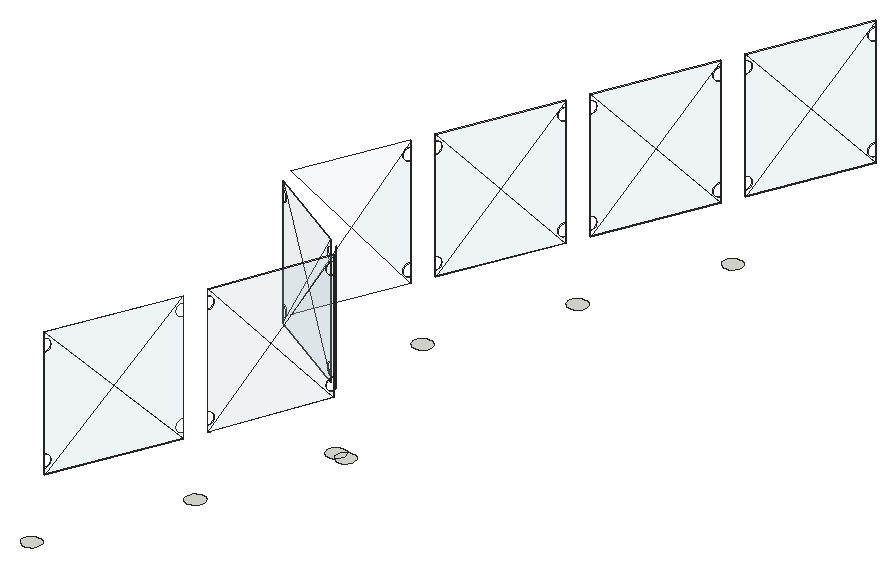
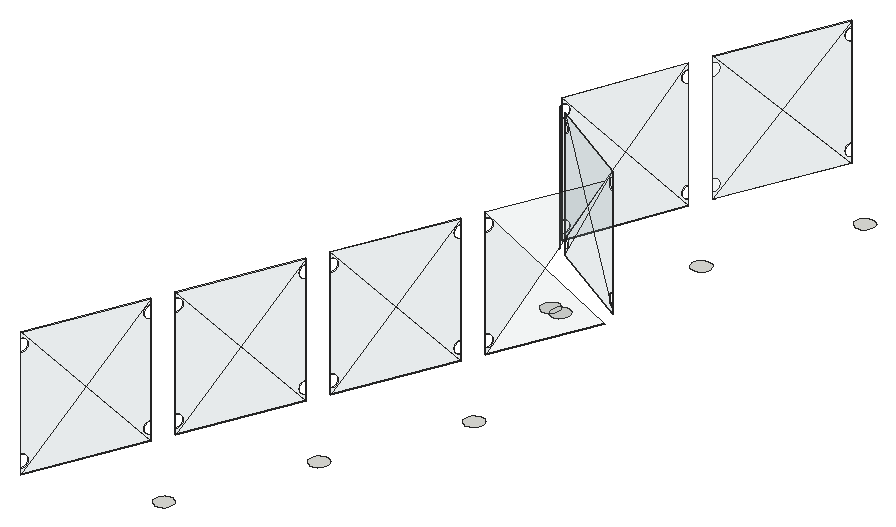
# SketchUp Ruby script. Lengths in inches.
U = 1.inch
M = Sketchup.active_model
def pt(a) = Geom::Point3d.new(a.map { |v| v * U })
def face(e, loops, mat)
  f = e.add_face(loops[0].map { |a| pt(a) })
  loops[1..].each { |l| e.add_face(l.map { |a| pt(a) }).erase! }
  f.material = f.back_material = mat if mat
  f
end
# faces: each face lists its corners as indices into pts; further lists are holes
def faces(e, pts, list, mat = nil) = list.each { |f| face(e, (f[0].is_a?(Array) ? f : [f]).map { |l| l.map { |i| pts[i] } }, mat) }
# xy, xz, yz: faces in a plane at the given z, y or x. An outline is a flat list of corners, or four numbers for a rectangle; further outlines are holes
def ring(l) = l.size == 4 ? [[l[0], l[1]], [l[2], l[1]], [l[2], l[3]], [l[0], l[3]]] : l.each_slice(2).to_a
def flat(e, list, mat, &to3) = list.each { |f| face(e, (f[0].is_a?(Array) ? f : [f]).map { |l| ring(l).map { |u, v| to3.(u, v) } }, mat) }
def xy(e, z, list, mat = nil) = flat(e, list, mat) { |x, y| [x, y, z] }
def xz(e, y, list, mat = nil) = flat(e, list, mat) { |x, z| [x, y, z] }
def yz(e, x, list, mat = nil) = flat(e, list, mat) { |y, z| [x, y, z] }
def lines(e, pts, list) = list.each { |a, b| e.add_line(pt(pts[a]), pt(pts[b])) }
# prism: a flat outline (further loops are holes) pulled along v
def prism(e, loops, v, mat = nil)
  f = face(e, loops, mat); d = Geom::Vector3d.new(v.map { |x| x * U })
  f.pushpull(f.normal.samedirection?(d) ? d.length : -d.length)
end
def box(e, o, s, mat = nil) = prism(e, [[o, [o[0] + s[0], o[1], o[2]], [o[0] + s[0], o[1] + s[1], o[2]], [o[0], o[1] + s[1], o[2]]]], [0, 0, s[2]], mat)
def at(x, y, z, deg = 0) = Geom::Transformation.translation(pt([x, y, z])) * Geom::Transformation.rotation(ORIGIN, Z_AXIS, deg.degrees)
def axes(o, x, y, z) = Geom::Transformation.new([*x, 0, *y, 0, *z, 0, *pt(o).to_a, 1])
def part(name) = M.definitions.add(name)
# library, detail: a bought-in or finely detailed component or shape, given as its bounding box
def library(name, o, s) = part(name).tap { |d| box(d.entities, o, s) }
def detail(e, o, s) = box(e.add_group.entities, o, s)
def put(e, d, t, mat = nil) = e.add_instance(d, t).tap { |i| i.material = mat if mat }
def group(e, t, mat = nil) = e.add_group.tap { |g| g.transformation = t; g.material = mat if mat }.entities
root = M.entities
M.materials.add("Glass_Safety_01").color = [204, 235, 244]
M.materials["Glass_Safety_01"].alpha = 0.1
xy(root,321.858,[[963.534,810.319,963.937,810.401,964.305,810.585,964.612,810.858,964.838,811.202,964.968,811.592,964.993,812.002,964.91,812.405,964.726,812.772,964.453,813.08,964.11,813.306,963.72,813.436,963.309,813.46,962.906,813.377,962.539,813.193,962.231,812.92,962.005,812.577,961.875,812.187,961.851,811.777,961.934,811.374,962.118,811.006,962.391,810.699,962.734,810.473,963.124,810.343],[973.7,833.66,974.103,833.743,974.471,833.927,974.778,834.2,975.004,834.543,975.134,834.933,975.159,835.344,975.076,835.746,974.892,836.114,974.619,836.421,974.276,836.648,973.886,836.777,973.475,836.802,973.072,836.719,972.705,836.535,972.397,836.262,972.171,835.919,972.041,835.529,972.017,835.118,972.1,834.716,972.284,834.348,972.557,834.041,972.9,833.814,973.29,833.685],[982.568,855.712,982.97,855.795,983.338,855.979,983.645,856.252,983.872,856.595,984.002,856.985,984.026,857.396,983.943,857.799,983.759,858.166,983.486,858.474,983.143,858.7,982.753,858.83,982.343,858.854,981.94,858.771,981.708,858.655,981.901,858.437,982.085,858.07,982.168,857.667,982.143,857.256,982.014,856.866,981.787,856.523,981.48,856.25,981.345,856.182,981.424,856.093,981.767,855.867,982.157,855.737],[980.71,855.983,981.112,856.066,981.345,856.182,981.151,856.4,980.967,856.768,980.884,857.171,980.909,857.581,981.039,857.971,981.265,858.314,981.572,858.587,981.708,858.655,981.628,858.745,981.285,858.971,980.895,859.101,980.485,859.125,980.082,859.042,979.714,858.858,979.407,858.585,979.18,858.242,979.051,857.852,979.026,857.442,979.109,857.039,979.293,856.671,979.566,856.364,979.909,856.138,980.299,856.008],[981.345,856.182,981.48,856.25,981.787,856.523,982.014,856.866,982.143,857.256,982.168,857.667,982.085,858.07,981.901,858.437,981.708,858.655,981.572,858.587,981.265,858.314,981.039,857.971,980.909,857.581,980.884,857.171,980.967,856.768,981.151,856.4],
  [970.873,887.274,971.276,887.357,971.644,887.541,971.951,887.814,972.177,888.157,972.307,888.547,972.332,888.957,972.249,889.36,972.065,889.728,971.792,890.035,971.449,890.261,971.059,890.391,970.648,890.416,970.245,890.333,969.878,890.149,969.57,889.876,969.344,889.533,969.214,889.143,969.19,888.732,969.273,888.33,969.457,887.962,969.73,887.655,970.073,887.428,970.463,887.298],[980.502,909.381,980.904,909.464,981.272,909.648,981.579,909.921,981.806,910.264,981.935,910.654,981.96,911.064,981.877,911.467,981.693,911.835,981.42,912.142,981.077,912.368,980.687,912.498,980.276,912.522,979.874,912.44,979.506,912.256,979.199,911.983,978.972,911.64,978.843,911.249,978.818,910.839,978.901,910.436,979.085,910.069,979.358,909.761,979.701,909.535,980.091,909.405],[990.144,931.521,990.547,931.604,990.915,931.788,991.222,932.061,991.448,932.404,991.578,932.794,991.602,933.204,991.52,933.607,991.336,933.975,991.063,934.282,990.72,934.508,990.329,934.638,989.919,934.663,989.516,934.58,989.149,934.396,988.841,934.123,988.615,933.78,988.485,933.39,988.461,932.979,988.544,932.577,988.728,932.209,989.001,931.901,989.344,931.675,989.734,931.545]])
xy(root,331.897,[[964.298,813.655,964.118,813.733,972.953,833.526],[964.118,813.733,972.772,833.605,972.953,833.526],[974.413,837.021,974.231,837.094,981.873,855.571],[974.231,837.094,981.69,855.645,981.873,855.571],[980.493,857.47,980.489,857.471,980.517,857.665],
  [980.493,857.47,980.517,857.665,980.521,857.665],[978.839,858.444,963.309,867.306,963.406,867.477],[978.839,858.444,963.406,867.477,978.936,858.615],[962.68,870.044,962.499,870.122,970.134,887.159],[962.499,870.122,969.953,887.238,970.134,887.159],
  [971.637,890.61,971.457,890.689,979.757,909.255],[971.457,890.689,979.577,909.334,979.757,909.255],[981.265,912.717,981.085,912.796,989.4,931.395],[981.085,912.796,989.219,931.473,989.4,931.395],[990.908,934.857,990.727,934.936,999.017,953.477],
  [990.727,934.936,998.837,953.555,999.017,953.477]],"Glass_Safety_01")
xz(root,857.665,[[980.517,331.897,980.521,333]],"Glass_Safety_01")
p = [[964.118,813.733,331.897],[964.298,813.655,331.897],[964.298,813.655,333],[964.298,813.655,335.126],[964.298,813.655,351.283],[964.298,813.655,353.409],
  [964.298,813.655,354.511],[964.118,813.733,354.511],[964.118,813.733,353.409],[964.118,813.733,351.283],[964.118,813.733,335.126],[964.118,813.733,333],
  [964.227,813.986,333.036],[964.33,814.221,333.142],[964.418,814.423,333.311],[964.485,814.577,333.531],[964.528,814.675,333.787],[964.542,814.708,334.0625],
  [964.528,814.675,334.338],[964.485,814.577,334.594],[964.418,814.423,334.814],[964.33,814.221,334.983],[964.227,813.986,335.089],[964.227,813.986,351.319],
  [964.33,814.221,351.425],[964.418,814.423,351.594],[964.485,814.577,351.814],[964.528,814.675,352.071],[964.542,814.708,352.346],[964.528,814.675,352.621],
  [964.485,814.577,352.877],[964.418,814.423,353.098],[964.33,814.221,353.267],[964.227,813.986,353.373],[972.772,833.605,331.897],[972.772,833.605,354.511],
  [972.772,833.605,353.409],[972.772,833.605,351.283],[972.772,833.605,335.126],[972.772,833.605,333],[964.408,813.907,335.089],[964.51,814.142,334.983],
  [964.598,814.344,334.814],[964.666,814.499,334.594],[964.708,814.596,334.338],[964.723,814.629,334.0625],[964.708,814.596,333.787],[964.666,814.499,333.531],
  [964.598,814.344,333.311],[964.51,814.142,333.142],[964.408,813.907,333.036],[972.953,833.526,354.511],[964.408,813.907,353.373],[964.51,814.142,353.267],
  [964.598,814.344,353.098],[964.666,814.499,352.877],[964.708,814.596,352.621],[964.723,814.629,352.346],[964.708,814.596,352.071],[964.666,814.499,351.814],
  [964.598,814.344,351.594],[964.51,814.142,351.425],[964.408,813.907,351.319],[972.953,833.526,331.897],[972.953,833.526,333],[972.892,833.387,333],
  [972.782,833.135,333.036],[972.68,832.9,333.142],[972.592,832.698,333.311],[972.524,832.543,333.531],[972.482,832.446,333.787],[972.467,832.412,334.0625],
  [972.482,832.446,334.338],[972.524,832.543,334.594],[972.592,832.698,334.814],[972.68,832.9,334.983],[972.782,833.135,335.089],[972.892,833.387,335.126],
  [972.953,833.526,335.126],[972.953,833.526,351.283],[972.892,833.387,351.283],[972.782,833.135,351.319],[972.68,832.9,351.425],[972.592,832.698,351.594],
  [972.524,832.543,351.814],[972.482,832.446,352.071],[972.467,832.412,352.346],[972.482,832.446,352.621],[972.524,832.543,352.877],[972.592,832.698,353.098],
  [972.68,832.9,353.267],[972.782,833.135,353.373],[972.892,833.387,353.409],[972.953,833.526,353.409],[974.231,837.094,331.897],[974.413,837.021,331.897],
  [974.413,837.021,333],[974.413,837.021,335.126],[974.413,837.021,351.283],[974.413,837.021,353.409],[974.413,837.021,354.511],[974.231,837.094,354.511],
  [974.231,837.094,353.409],[974.231,837.094,351.283],[974.231,837.094,335.126],[974.231,837.094,333],[974.516,837.276,335.089],[974.612,837.514,334.983],
  [974.694,837.718,334.814],[974.757,837.875,334.594],[974.797,837.973,334.338],[974.81,838.007,334.0625],[974.797,837.973,333.787],[974.757,837.875,333.531],
  [974.694,837.718,333.311],[974.612,837.514,333.142],[974.516,837.276,333.036],[981.873,855.571,354.511],[974.516,837.276,353.373],[974.612,837.514,353.267],
  [974.694,837.718,353.098],[974.757,837.875,352.877],[974.797,837.973,352.621],[974.81,838.007,352.346],[974.797,837.973,352.071],[974.757,837.875,351.814],
  [974.694,837.718,351.594],[974.612,837.514,351.425],[974.516,837.276,351.319],[981.873,855.571,331.897],[981.873,855.571,333],[981.812,855.42,333],
  [981.709,855.165,333.036],[981.614,854.927,333.142],[981.532,854.723,333.311],[981.469,854.566,333.531],[981.429,854.468,333.787],[981.415,854.434,334.0625],
  [981.429,854.468,334.338],[981.469,854.566,334.594],[981.532,854.723,334.814],[981.614,854.927,334.983],[981.709,855.165,335.089],[981.812,855.42,335.126],
  [981.873,855.571,335.126],[981.873,855.571,351.283],[981.812,855.42,351.283],[981.709,855.165,351.319],[981.614,854.927,351.425],[981.532,854.723,351.594],
  [981.469,854.566,351.814],[981.429,854.468,352.071],[981.415,854.434,352.346],[981.429,854.468,352.621],[981.469,854.566,352.877],[981.532,854.723,353.098],
  [981.614,854.927,353.267],[981.709,855.165,353.373],[981.812,855.42,353.409],[981.873,855.571,353.409],[974.333,837.349,333.036],[974.429,837.587,333.142],
  [974.511,837.791,333.311],[974.574,837.948,333.531],[974.614,838.047,333.787],[974.627,838.08,334.0625],[974.614,838.047,334.338],[974.574,837.948,334.594],
  [974.511,837.791,334.814],[974.429,837.587,334.983],[974.333,837.349,335.089],[974.333,837.349,351.319],[974.429,837.587,351.425],[974.511,837.791,351.594],
  [974.574,837.948,351.814],[974.614,838.047,352.071],[974.627,838.08,352.346],[974.614,838.047,352.621],[974.574,837.948,352.877],[974.511,837.791,353.098],
  [974.429,837.587,353.267],[974.333,837.349,353.373],[981.69,855.645,331.897],[981.69,855.645,351.283],[981.69,855.645,335.126],[981.629,855.494,335.126],
  [981.527,855.238,335.089],[981.431,855,334.983],[981.349,854.796,334.814],[981.286,854.639,334.594],[981.246,854.541,334.338],[981.233,854.507,334.0625],
  [981.246,854.541,333.787],[981.286,854.639,333.531],[981.349,854.796,333.311],[981.431,855,333.142],[981.527,855.238,333.036],[981.629,855.494,333],
  [981.69,855.645,333],[981.69,855.645,354.511],[981.69,855.645,353.409],[981.629,855.494,353.409],[981.527,855.238,353.373],[981.431,855,353.267],
  [981.349,854.796,353.098],[981.286,854.639,352.877],[981.246,854.541,352.621],[981.233,854.507,352.346],[981.246,854.541,352.071],[981.286,854.639,351.814],
  [981.349,854.796,351.594],[981.431,855,351.425],[981.527,855.238,351.319],[981.629,855.494,351.283],[980.493,857.47,331.897],[980.493,857.47,333],
  [980.489,857.471,333],[980.489,857.471,331.897],[980.521,857.665,331.897],[980.521,857.665,333],[980.521,857.665,335.126],[980.521,857.665,351.283],
  [980.521,857.665,353.409],[980.521,857.665,354.511],[980.493,857.47,354.511],[980.493,857.47,353.409],[980.493,857.47,351.283],[980.493,857.47,335.126],
  [980.517,857.665,331.897],[980.489,857.471,335.125],[980.489,857.471,351.284],[980.489,857.471,353.408],[980.489,857.471,354.511],[980.517,857.665,354.511],
  [980.517,857.665,353.408],[980.517,857.665,351.284],[980.517,857.665,335.125],[980.517,857.665,333],[978.839,858.444,331.897],[978.839,858.444,333],
  [978.6,858.581,333.036],[978.377,858.708,333.142],[978.186,858.817,333.311],[978.039,858.901,333.531],[977.947,858.953,333.787],[977.915,858.971,334.0625],
  [977.947,858.953,334.338],[978.039,858.901,334.594],[978.186,858.817,334.814],[978.377,858.708,334.983],[978.6,858.581,335.089],[978.839,858.444,335.126],
  [978.839,858.444,351.283],[978.6,858.581,351.319],[978.377,858.708,351.425],[978.186,858.817,351.594],[978.039,858.901,351.814],[977.947,858.953,352.071],
  [977.915,858.971,352.346],[977.947,858.953,352.621],[978.039,858.901,352.877],[978.186,858.817,353.098],[978.377,858.708,353.267],[978.6,858.581,353.373],
  [978.839,858.444,353.409],[978.839,858.444,354.511],[963.309,867.306,331.897],[963.309,867.306,351.283],[963.309,867.306,335.126],[963.464,867.217,335.126],
  [963.703,867.081,335.089],[963.926,866.954,334.983],[964.117,866.845,334.814],[964.264,866.761,334.594],[964.356,866.708,334.338],[964.388,866.69,334.0625],
  [964.356,866.708,333.787],[964.264,866.761,333.531],[964.117,866.845,333.311],[963.926,866.954,333.142],[963.703,867.081,333.036],[963.464,867.217,333],
  [963.309,867.306,333],[963.309,867.306,354.511],[963.309,867.306,353.409],[963.464,867.217,353.409],[963.703,867.081,353.373],[963.926,866.954,353.267],
  [964.117,866.845,353.098],[964.264,866.761,352.877],[964.356,866.708,352.621],[964.388,866.69,352.346],[964.356,866.708,352.071],[964.264,866.761,351.814],
  [964.117,866.845,351.594],[963.926,866.954,351.425],[963.703,867.081,351.319],[963.464,867.217,351.283],[978.936,858.615,331.897],[978.936,858.615,333],
  [978.936,858.615,335.126],[978.936,858.615,351.283],[978.936,858.615,353.409],[978.936,858.615,354.511],[978.697,858.752,335.089],[978.475,858.879,334.983],
  [978.283,858.988,334.814],[978.137,859.072,334.594],[978.044,859.124,334.338],[978.013,859.142,334.0625],[978.044,859.124,333.787],[978.137,859.072,333.531],
  [978.283,858.988,333.311],[978.475,858.879,333.142],[978.697,858.752,333.036],[963.406,867.477,354.511],[978.697,858.752,353.373],[978.475,858.879,353.267],
  [978.283,858.988,353.098],[978.137,859.072,352.877],[978.044,859.124,352.621],[978.013,859.142,352.346],[978.044,859.124,352.071],[978.137,859.072,351.814],
  [978.283,858.988,351.594],[978.475,858.879,351.425],[978.697,858.752,351.319],[963.406,867.477,331.897],[963.406,867.477,333],[963.562,867.388,333],
  [963.801,867.252,333.036],[964.024,867.125,333.142],[964.215,867.016,333.311],[964.361,866.932,333.531],[964.454,866.879,333.787],[964.485,866.861,334.0625],
  [964.454,866.879,334.338],[964.361,866.932,334.594],[964.215,867.016,334.814],[964.024,867.125,334.983],[963.801,867.252,335.089],[963.562,867.388,335.126],
  [963.406,867.477,335.126],[963.406,867.477,351.283],[963.562,867.388,351.283],[963.801,867.252,351.319],[964.024,867.125,351.425],[964.215,867.016,351.594],
  [964.361,866.932,351.814],[964.454,866.879,352.071],[964.485,866.861,352.346],[964.454,866.879,352.621],[964.361,866.932,352.877],[964.215,867.016,353.098],
  [964.024,867.125,353.267],[963.801,867.252,353.373],[963.562,867.388,353.409],[963.406,867.477,353.409],[970.134,887.159,331.897],[970.134,887.159,333],
  [970.065,887.001,333],[969.955,886.749,333.036],[969.853,886.514,333.142],[969.765,886.312,333.311],[969.697,886.157,333.531],[969.655,886.059,333.787],
  [969.641,886.026,334.0625],[969.655,886.059,334.338],[969.697,886.157,334.594],[969.765,886.312,334.814],[969.853,886.514,334.983],[969.955,886.749,335.089],
  [970.065,887.001,335.126],[970.134,887.159,335.126],[970.134,887.159,351.283],[970.065,887.001,351.283],[969.955,886.749,351.319],[969.853,886.514,351.425],
  [969.765,886.312,351.594],[969.697,886.157,351.814],[969.655,886.059,352.071],[969.641,886.026,352.346],[969.655,886.059,352.621],[969.697,886.157,352.877],
  [969.765,886.312,353.098],[969.853,886.514,353.267],[969.955,886.749,353.373],[970.065,887.001,353.409],[970.134,887.159,353.409],[970.134,887.159,354.511],
  [962.68,870.044,331.897],[969.953,887.238,351.283],[969.953,887.238,335.126],[969.884,887.079,335.126],[969.775,886.827,335.089],[969.672,886.592,334.983],
  [969.584,886.39,334.814],[969.517,886.235,334.594],[969.474,886.138,334.338],[969.46,886.105,334.0625],[969.474,886.138,333.787],[969.517,886.235,333.531],
  [969.584,886.39,333.311],[969.672,886.592,333.142],[969.775,886.827,333.036],[969.884,887.079,333],[969.953,887.238,333],[969.953,887.238,331.897],
  [962.499,870.122,354.511],[969.953,887.238,354.511],[969.953,887.238,353.409],[969.884,887.079,353.409],[969.775,886.827,353.373],[969.672,886.592,353.267],
  [969.584,886.39,353.098],[969.517,886.235,352.877],[969.474,886.138,352.621],[969.46,886.105,352.346],[969.474,886.138,352.071],[969.517,886.235,351.814],
  [969.584,886.39,351.594],[969.672,886.592,351.425],[969.775,886.827,351.319],[969.884,887.079,351.283],[971.457,890.689,331.897],[971.637,890.61,331.897],
  [971.637,890.61,333],[971.637,890.61,335.126],[971.637,890.61,351.283],[971.637,890.61,353.409],[971.637,890.61,354.511],[971.457,890.689,354.511],
  [971.457,890.689,353.409],[971.457,890.689,351.283],[971.457,890.689,335.126],[971.457,890.689,333],[971.747,890.863,335.089],[971.849,891.098,334.983],
  [971.937,891.299,334.814],[972.005,891.454,334.594],[972.047,891.552,334.338],[972.061,891.585,334.0625],[972.047,891.552,333.787],[972.005,891.454,333.531],
  [971.937,891.299,333.311],[971.849,891.098,333.142],[971.747,890.863,333.036],[979.757,909.255,354.511],[971.747,890.863,353.373],[971.849,891.098,353.267],
  [971.937,891.299,353.098],[972.005,891.454,352.877],[972.047,891.552,352.621],[972.061,891.585,352.346],[972.047,891.552,352.071],[972.005,891.454,351.814],
  [971.937,891.299,351.594],[971.849,891.098,351.425],[971.747,890.863,351.319],[979.757,909.255,331.897],[979.757,909.255,333],[979.693,909.108,333],
  [979.583,908.855,333.036],[979.481,908.62,333.142],[979.393,908.418,333.311],[979.326,908.264,333.531],[979.283,908.166,333.787],[979.269,908.133,334.0625],
  [979.283,908.166,334.338],[979.326,908.264,334.594],[979.393,908.418,334.814],[979.481,908.62,334.983],[979.583,908.855,335.089],[979.693,909.108,335.126],
  [979.757,909.255,335.126],[979.757,909.255,351.283],[979.693,909.108,351.283],[979.583,908.855,351.319],[979.481,908.62,351.425],[979.393,908.418,351.594],
  [979.326,908.264,351.814],[979.283,908.166,352.071],[979.269,908.133,352.346],[979.283,908.166,352.621],[979.326,908.264,352.877],[979.393,908.418,353.098],
  [979.481,908.62,353.267],[979.583,908.855,353.373],[979.693,909.108,353.409],[979.757,909.255,353.409],[971.566,890.941,333.036],[971.669,891.176,333.142],
  [971.757,891.378,333.311],[971.824,891.533,333.531],[971.867,891.63,333.787],[971.881,891.663,334.0625],[971.867,891.63,334.338],[971.824,891.533,334.594],
  [971.757,891.378,334.814],[971.669,891.176,334.983],[971.566,890.941,335.089],[971.566,890.941,351.319],[971.669,891.176,351.425],[971.757,891.378,351.594],
  [971.824,891.533,351.814],[971.867,891.63,352.071],[971.881,891.663,352.346],[971.867,891.63,352.621],[971.824,891.533,352.877],[971.757,891.378,353.098],
  [971.669,891.176,353.267],[971.566,890.941,353.373],[979.577,909.334,331.897],[979.577,909.334,351.283],[979.577,909.334,335.126],[979.513,909.186,335.126],
  [979.403,908.934,335.089],[979.3,908.699,334.983],[979.213,908.497,334.814],[979.145,908.342,334.594],[979.103,908.245,334.338],[979.088,908.212,334.0625],
  [979.103,908.245,333.787],[979.145,908.342,333.531],[979.213,908.497,333.311],[979.3,908.699,333.142],[979.403,908.934,333.036],[979.513,909.186,333],
  [979.577,909.334,333],[979.577,909.334,354.511],[979.577,909.334,353.409],[979.513,909.186,353.409],[979.403,908.934,353.373],[979.3,908.699,353.267],
  [979.213,908.497,353.098],[979.145,908.342,352.877],[979.103,908.245,352.621],[979.088,908.212,352.346],[979.103,908.245,352.071],[979.145,908.342,351.814],
  [979.213,908.497,351.594],[979.3,908.699,351.425],[979.403,908.934,351.319],[979.513,909.186,351.283],[981.085,912.796,331.897],[981.265,912.717,331.897],
  [981.265,912.717,333],[981.265,912.717,335.126],[981.265,912.717,351.283],[981.265,912.717,353.409],[981.265,912.717,354.511],[981.085,912.796,354.511],
  [981.085,912.796,353.409],[981.085,912.796,351.283],[981.085,912.796,335.126],[981.085,912.796,333],[981.375,912.969,335.089],[981.477,913.204,334.983],
  [981.565,913.406,334.814],[981.633,913.561,334.594],[981.675,913.658,334.338],[981.69,913.692,334.0625],[981.675,913.658,333.787],[981.633,913.561,333.531],
  [981.565,913.406,333.311],[981.477,913.204,333.142],[981.375,912.969,333.036],[989.4,931.395,354.511],[981.375,912.969,353.373],[981.477,913.204,353.267],
  [981.565,913.406,353.098],[981.633,913.561,352.877],[981.675,913.658,352.621],[981.69,913.692,352.346],[981.675,913.658,352.071],[981.633,913.561,351.814],
  [981.565,913.406,351.594],[981.477,913.204,351.425],[981.375,912.969,351.319],[989.4,931.395,331.897],[989.4,931.395,333],[989.336,931.248,333],
  [989.226,930.996,333.036],[989.124,930.76,333.142],[989.036,930.559,333.311],[988.968,930.404,333.531],[988.926,930.306,333.787],[988.911,930.273,334.0625],
  [988.926,930.306,334.338],[988.968,930.404,334.594],[989.036,930.559,334.814],[989.124,930.76,334.983],[989.226,930.996,335.089],[989.336,931.248,335.126],
  [989.4,931.395,335.126],[989.4,931.395,351.283],[989.336,931.248,351.283],[989.226,930.996,351.319],[989.124,930.76,351.425],[989.036,930.559,351.594],
  [988.968,930.404,351.814],[988.926,930.306,352.071],[988.911,930.273,352.346],[988.926,930.306,352.621],[988.968,930.404,352.877],[989.036,930.559,353.098],
  [989.124,930.76,353.267],[989.226,930.996,353.373],[989.336,931.248,353.409],[989.4,931.395,353.409],[981.195,913.048,333.036],[981.297,913.283,333.142],
  [981.385,913.485,333.311],[981.452,913.64,333.531],[981.495,913.737,333.787],[981.509,913.77,334.0625],[981.495,913.737,334.338],[981.452,913.64,334.594],
  [981.385,913.485,334.814],[981.297,913.283,334.983],[981.195,913.048,335.089],[981.195,913.048,351.319],[981.297,913.283,351.425],[981.385,913.485,351.594],
  [981.452,913.64,351.814],[981.495,913.737,352.071],[981.509,913.77,352.346],[981.495,913.737,352.621],[981.452,913.64,352.877],[981.385,913.485,353.098],
  [981.297,913.283,353.267],[981.195,913.048,353.373],[989.219,931.473,331.897],[989.219,931.473,351.283],[989.219,931.473,335.126],[989.155,931.326,335.126],
  [989.046,931.074,335.089],[988.943,930.839,334.983],[988.855,930.637,334.814],[988.788,930.482,334.594],[988.745,930.385,334.338],[988.731,930.352,334.0625],
  [988.745,930.385,333.787],[988.788,930.482,333.531],[988.855,930.637,333.311],[988.943,930.839,333.142],[989.046,931.074,333.036],[989.155,931.326,333],
  [989.219,931.473,333],[989.219,931.473,354.511],[989.219,931.473,353.409],[989.155,931.326,353.409],[989.046,931.074,353.373],[988.943,930.839,353.267],
  [988.855,930.637,353.098],[988.788,930.482,352.877],[988.745,930.385,352.621],[988.731,930.352,352.346],[988.745,930.385,352.071],[988.788,930.482,351.814],
  [988.855,930.637,351.594],[988.943,930.839,351.425],[989.046,931.074,351.319],[989.155,931.326,351.283],[990.727,934.936,331.897],[990.908,934.857,331.897],
  [990.908,934.857,333],[990.908,934.857,335.126],[990.908,934.857,351.283],[990.908,934.857,353.409],[990.908,934.857,354.511],[990.727,934.936,354.511],
  [990.727,934.936,353.409],[990.727,934.936,351.283],[990.727,934.936,335.126],[990.727,934.936,333],[990.837,935.188,333.036],[990.94,935.423,333.142],
  [991.028,935.625,333.311],[991.095,935.78,333.531],[991.137,935.877,333.787],[991.152,935.91,334.0625],[991.137,935.877,334.338],[991.095,935.78,334.594],
  [991.028,935.625,334.814],[990.94,935.423,334.983],[990.837,935.188,335.089],[990.837,935.188,351.319],[990.94,935.423,351.425],[991.028,935.625,351.594],
  [991.095,935.78,351.814],[991.137,935.877,352.071],[991.152,935.91,352.346],[991.137,935.877,352.621],[991.095,935.78,352.877],[991.028,935.625,353.098],
  [990.94,935.423,353.267],[990.837,935.188,353.373],[998.837,953.555,331.897],[998.837,953.555,351.283],[998.837,953.555,335.125],[998.772,953.408,335.125],
  [998.663,953.155,335.089],[998.56,952.92,334.983],[998.472,952.718,334.814],[998.405,952.564,334.594],[998.362,952.466,334.338],[998.348,952.433,334.0625],
  [998.362,952.466,333.787],[998.405,952.564,333.531],[998.472,952.718,333.311],[998.56,952.92,333.142],[998.663,953.155,333.036],[998.772,953.408,333],
  [998.837,953.555,333],[998.837,953.555,354.511],[998.837,953.555,353.409],[998.772,953.408,353.409],[998.663,953.155,353.373],[998.56,952.92,353.267],
  [998.472,952.718,353.098],[998.405,952.564,352.877],[998.362,952.466,352.621],[998.348,952.433,352.346],[998.362,952.466,352.071],[998.405,952.564,351.814],
  [998.472,952.718,351.594],[998.56,952.92,351.425],[998.663,953.155,351.319],[998.772,953.408,351.283],[991.018,935.11,335.089],[991.12,935.345,334.983],
  [991.208,935.546,334.814],[991.275,935.701,334.594],[991.318,935.799,334.338],[991.332,935.832,334.0625],[991.318,935.799,333.787],[991.275,935.701,333.531],
  [991.208,935.546,333.311],[991.12,935.345,333.142],[991.018,935.11,333.036],[999.017,953.477,354.511],[991.018,935.11,353.373],[991.12,935.345,353.267],
  [991.208,935.546,353.098],[991.275,935.701,352.877],[991.318,935.799,352.621],[991.332,935.832,352.346],[991.318,935.799,352.071],[991.275,935.701,351.814],
  [991.208,935.546,351.594],[991.12,935.345,351.425],[991.018,935.11,351.319],[999.017,953.477,331.897],[999.017,953.477,333],[998.953,953.329,333],
  [998.843,953.077,333.036],[998.741,952.842,333.142],[998.653,952.64,333.311],[998.585,952.485,333.531],[998.543,952.388,333.787],[998.528,952.354,334.0625],
  [998.543,952.388,334.338],[998.585,952.485,334.594],[998.653,952.64,334.814],[998.741,952.842,334.983],[998.843,953.077,335.089],[998.953,953.329,335.125],
  [999.017,953.477,335.125],[999.017,953.477,351.283],[998.953,953.329,351.283],[998.843,953.077,351.319],[998.741,952.842,351.425],[998.653,952.64,351.594],
  [998.585,952.485,351.814],[998.543,952.388,352.071],[998.528,952.354,352.346],[998.543,952.388,352.621],[998.585,952.485,352.877],[998.653,952.64,353.098],
  [998.741,952.842,353.267],[998.843,953.077,353.373],[998.953,953.329,353.409],[999.017,953.477,353.409]]
faces(root,p,[[0,1,2,3,4,5,6,7,8,9,10,11],[0,11,12,13,14,15,16,17,18,19,20,21,22,10,9,23,24,25,26,27,28,29,30,31,32,33,8,7,34],[34,7,35,36,37,38,39],[4,3,40,41,42,43,44,45,46,47,48,49,50,2,1,51,6,5,52,53,54,55,56,57,58,59,60,61,62],[63,64,65,66,67,68,69,70,71,72,73,74,75,76,77,78,79,80,81,82,83,84,85,86,87,88,89,90,91,92,93,51,1],[63,34,39,38,37,36,35,51,93,79,78,64],[94,95,96,97,98,99,100,101,102,103,104,105],[98,97,106,107,108,109,110,111,112,113,114,115,116,96,95,117,100,99,118,119,120,121,122,123,124,125,126,127,128],
  [129,130,131,132,133,134,135,136,137,138,139,140,141,142,143,144,145,146,147,148,149,150,151,152,153,154,155,156,157,158,159,117,95],[94,105,160,161,162,163,164,165,166,167,168,169,170,104,103,171,172,173,174,175,176,177,178,179,180,181,102,101,182],[183,184,185,186,187,188,189,190,191,192,193,194,195,196,197,198,182,101,199,200,201,202,203,204,205,206,207,208,209,210,211,212,213],[129,182,198,184,183,200,199,117,159,145,144,130],[214,215,216,217],[214,218,219,220,221,222,223,224,225,226,227,215],[228,217,216,229,230,231,232,233,234,235,236,237],[238,239,240,241,242,243,244,245,246,247,248,249,250,251,252,253,254,255,256,257,258,259,260,261,262,263,264,265,266],
  [267,268,269,270,271,272,273,274,275,276,277,278,279,280,281,282,266,265,283,284,285,286,287,288,289,290,291,292,293,294,295,296,297],[238,298,299,300,301,302,303,265,264,252,251,239],[301,300,304,305,306,307,308,309,310,311,312,313,314,299,298,315,303,302,316,317,318,319,320,321,322,323,324,325,326],[327,328,329,330,331,332,333,334,335,336,337,338,339,340,341,342,343,344,345,346,347,348,349,350,351,352,353,354,355,356,357,315,298],[327,266,282,268,267,284,283,315,357,343,342,328],[358,359,360,361,362,363,364,365,366,367,368,369,370,371,372,373,374,375,376,377,378,379,380,381,382,383,384,385,386,387,388,389,390],[391,392,393,394,395,396,397,398,399,400,401,402,403,404,405,406,407,408,409,410,411,412,413,414,415,416,417,418,419,420,421,422,423],[358,407,406,392,391,410,409,389,388,374,373,359],
  [424,425,426,427,428,429,430,431,432,433,434,435],[428,427,436,437,438,439,440,441,442,443,444,445,446,426,425,447,430,429,448,449,450,451,452,453,454,455,456,457,458],[459,460,461,462,463,464,465,466,467,468,469,470,471,472,473,474,475,476,477,478,479,480,481,482,483,484,485,486,487,488,489,447,425],[424,435,490,491,492,493,494,495,496,497,498,499,500,434,433,501,502,503,504,505,506,507,508,509,510,511,432,431,512],[513,514,515,516,517,518,519,520,521,522,523,524,525,526,527,528,512,431,529,530,531,532,533,534,535,536,537,538,539,540,541,542,543],[459,512,528,514,513,530,529,447,489,475,474,460],[544,545,546,547,548,549,550,551,552,553,554,555],[548,547,556,557,558,559,560,561,562,563,564,565,566,546,545,567,550,549,568,569,570,571,572,573,574,575,576,577,578],
  [579,580,581,582,583,584,585,586,587,588,589,590,591,592,593,594,595,596,597,598,599,600,601,602,603,604,605,606,607,608,609,567,545],[544,555,610,611,612,613,614,615,616,617,618,619,620,554,553,621,622,623,624,625,626,627,628,629,630,631,552,551,632],[633,634,635,636,637,638,639,640,641,642,643,644,645,646,647,648,632,551,649,650,651,652,653,654,655,656,657,658,659,660,661,662,663],[579,632,648,634,633,650,649,567,609,595,594,580],[664,665,666,667,668,669,670,671,672,673,674,675],[664,675,676,677,678,679,680,681,682,683,684,685,686,674,673,687,688,689,690,691,692,693,694,695,696,697,672,671,698],[699,700,701,702,703,704,705,706,707,708,709,710,711,712,713,714,698,671,715,716,717,718,719,720,721,722,723,724,725,726,727,728,729],[668,667,730,731,732,733,734,735,736,737,738,739,740,666,665,741,670,669,742,743,744,745,746,747,748,749,750,751,752],
  [753,754,755,756,757,758,759,760,761,762,763,764,765,766,767,768,769,770,771,772,773,774,775,776,777,778,779,780,781,782,783,741,665],[753,698,714,700,699,716,715,741,783,769,768,754]],"Glass_Safety_01")
